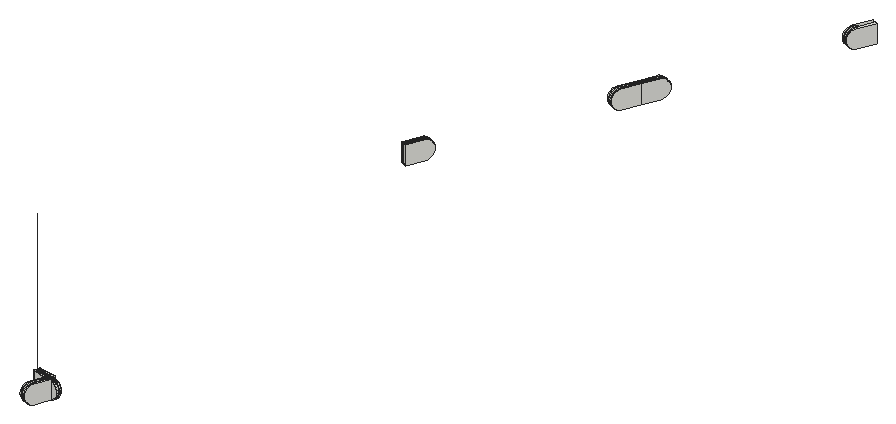
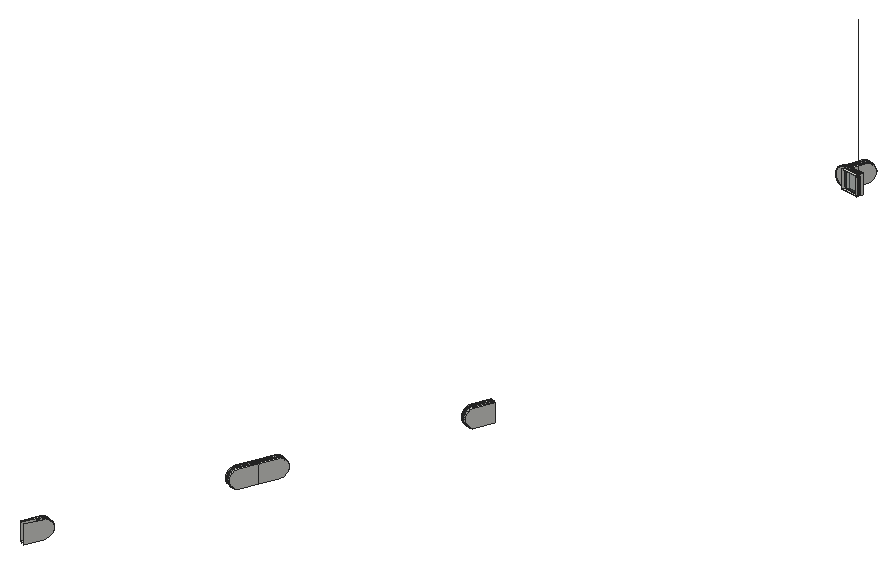
# SketchUp Ruby script. Lengths in inches.
U = 1.inch
M = Sketchup.active_model
def pt(a) = Geom::Point3d.new(a.map { |v| v * U })
def face(e, loops, mat)
  f = e.add_face(loops[0].map { |a| pt(a) })
  loops[1..].each { |l| e.add_face(l.map { |a| pt(a) }).erase! }
  f.material = f.back_material = mat if mat
  f
end
# faces: each face lists its corners as indices into pts; further lists are holes
def faces(e, pts, list, mat = nil) = list.each { |f| face(e, (f[0].is_a?(Array) ? f : [f]).map { |l| l.map { |i| pts[i] } }, mat) }
# xy, xz, yz: faces in a plane at the given z, y or x. An outline is a flat list of corners, or four numbers for a rectangle; further outlines are holes
def ring(l) = l.size == 4 ? [[l[0], l[1]], [l[2], l[1]], [l[2], l[3]], [l[0], l[3]]] : l.each_slice(2).to_a
def flat(e, list, mat, &to3) = list.each { |f| face(e, (f[0].is_a?(Array) ? f : [f]).map { |l| ring(l).map { |u, v| to3.(u, v) } }, mat) }
def xy(e, z, list, mat = nil) = flat(e, list, mat) { |x, y| [x, y, z] }
def xz(e, y, list, mat = nil) = flat(e, list, mat) { |x, z| [x, y, z] }
def yz(e, x, list, mat = nil) = flat(e, list, mat) { |y, z| [x, y, z] }
def lines(e, pts, list) = list.each { |a, b| e.add_line(pt(pts[a]), pt(pts[b])) }
# prism: a flat outline (further loops are holes) pulled along v
def prism(e, loops, v, mat = nil)
  f = face(e, loops, mat); d = Geom::Vector3d.new(v.map { |x| x * U })
  f.pushpull(f.normal.samedirection?(d) ? d.length : -d.length)
end
def box(e, o, s, mat = nil) = prism(e, [[o, [o[0] + s[0], o[1], o[2]], [o[0] + s[0], o[1] + s[1], o[2]], [o[0], o[1] + s[1], o[2]]]], [0, 0, s[2]], mat)
def at(x, y, z, deg = 0) = Geom::Transformation.translation(pt([x, y, z])) * Geom::Transformation.rotation(ORIGIN, Z_AXIS, deg.degrees)
def axes(o, x, y, z) = Geom::Transformation.new([*x, 0, *y, 0, *z, 0, *pt(o).to_a, 1])
def part(name) = M.definitions.add(name)
# library, detail: a bought-in or finely detailed component or shape, given as its bounding box
def library(name, o, s) = part(name).tap { |d| box(d.entities, o, s) }
def detail(e, o, s) = box(e.add_group.entities, o, s)
def put(e, d, t, mat = nil) = e.add_instance(d, t).tap { |i| i.material = mat if mat }
def group(e, t, mat = nil) = e.add_group.tap { |g| g.transformation = t; g.material = mat if mat }.entities
root = M.entities
M.materials.add("Glass_Safety_01").color = [204, 235, 244]
M.materials["Glass_Safety_01"].alpha = 0.1
xy(root,333,[[982.07,855.32,981.8125,855.42,981.87,855.57,982.41,856.91,982.49,856.9,982.52,857.09,982.53,857.17,982.54,857.23,982.55,857.25,982.8,857.14],[981.63,855.49,981.375,855.6,981.93,856.98,982.21,856.94],[982.49,856.9,982.41,856.91,982.49,857.1,982.52,857.09],[982.4,856.91,982.21,856.94,982.29,857.13,982.43,857.11],[982.4,856.91,982.43,857.11,982.49,857.1,982.41,856.91],
  [982.21,856.94,981.93,856.98,982.01,857.17,982.29,857.13],[981.93,856.98,980.54,857.18,980.57,857.38,982.01,857.17],[982.52,857.09,982.49,857.1,982.52,857.17,982.53,857.17],[982.49,857.1,982.43,857.11,982.44,857.1875,982.52,857.17],[982.43,857.11,982.29,857.13,982.32,857.2,982.44,857.1875],
  [982.29,857.13,982.01,857.17,982.04,857.24,982.32,857.2],[982.01,857.17,980.57,857.38,980.58,857.46,982.04,857.24],[982.52,857.17,982.44,857.1875,982.32,857.2,982.36,857.32,982.11,857.42,982.04,857.24,980.58,857.46,980.61,857.65,980.63,857.65,980.65,857.64,980.65,857.65,982.47,857.38,982.56,857.37,982.54,857.23],[982.52,857.17,982.54,857.23,982.53,857.17],[980.54,857.18,980.45,857.2,980.47,857.34,980.54,857.46,980.58,857.46,980.57,857.38],
  [982.32,857.2,982.04,857.24,982.11,857.42,982.36,857.32],[980.47,857.34,980.49,857.47,980.54,857.46],[982.47,857.38,980.65,857.65,980.78,857.88,980.72,857.91,982.51,857.65],[980.65,857.64,980.63,857.65,980.65,857.65],[980.61,857.65,980.52,857.66,980.53,857.71,980.63,857.65],
  [980.63,857.65,980.53,857.71,980.5625,857.9375,980.72,857.91,980.78,857.88,980.65,857.65],[980.73,910.8,980.48,910.91,981.27,912.72,981.52,912.61],[980.3,910.99,980.05,911.1,980.83,912.91,981.08,912.8],[989.59,931.14,989.34,931.25,989.4,931.39,990.12,933.05,990.375,932.94],[989.16,931.33,988.9,931.4375,989.6875,933.24,989.94,933.13,989.22,931.47],
  [990.375,932.94,990.12,933.05,990.91,934.86,991.16,934.75],[989.94,933.13,989.6875,933.24,990.47,935.05,990.73,934.9375],[999.21,953.22,998.95,953.33,999.02,953.48,999.74,955.13,999.99,955.02]])
xy(root,333.08,[[981.96,855.79,981.78,855.86,982.32,857.2,982.44,857.1875,982.46,857.28,982.55,857.25],[982.44,857.1875,982.32,857.2,982.36,857.32,982.46,857.28],[982.32,857.2,982.14,857.23,982.17,857.42,982.47,857.38,982.46,857.28,982.36,857.32],[982.14,857.23,980.88,857.41,980.91,857.61,982.17,857.42],[980.88,857.41,980.58,857.46,980.6,857.55,980.65,857.64,980.63,857.65,980.91,857.61],
  [980.6,857.55,980.61,857.65,980.63,857.65,980.65,857.64],[980.48,910.91,980.3,910.99,980.93,912.43,981.11,912.36],[989.49,931.61,989.3125,931.6875,989.94,933.13,990.12,933.05],[990.12,933.05,989.94,933.13,990.57,934.57,990.75,934.5]],"Glass_Safety_01")
xy(root,335.05,[[981.96,855.79,982.55,857.25,982.46,857.28,982.44,857.1875,982.32,857.2,981.78,855.86],[982.44,857.1875,982.46,857.28,982.36,857.32,982.32,857.2],[982.32,857.2,982.36,857.32,982.46,857.28,982.47,857.38,982.17,857.42,982.14,857.23],[982.14,857.23,982.17,857.42,980.91,857.61,980.88,857.41],[980.88,857.41,980.91,857.61,980.63,857.65,980.65,857.64,980.6,857.55,980.58,857.46],
  [980.6,857.55,980.65,857.64,980.63,857.65,980.61,857.65],[980.48,910.91,981.11,912.36,980.93,912.43,980.3,910.99],[989.49,931.61,990.12,933.05,989.94,933.13,989.3125,931.6875],[990.12,933.05,990.75,934.5,990.57,934.57,989.94,933.13]],"Glass_Safety_01")
xy(root,335.125,[[982.07,855.32,982.8,857.14,982.55,857.25,982.54,857.23,982.53,857.17,982.52,857.09,982.49,856.9,982.41,856.91,981.87,855.57,981.8125,855.42],[981.63,855.49,982.21,856.94,981.93,856.98,981.375,855.6],[982.49,856.9,982.52,857.09,982.49,857.1,982.41,856.91],[982.4,856.91,982.43,857.11,982.29,857.13,982.21,856.94],[982.4,856.91,982.41,856.91,982.49,857.1,982.43,857.11],
  [982.21,856.94,982.29,857.13,982.01,857.17,981.93,856.98],[981.93,856.98,982.01,857.17,980.57,857.38,980.54,857.18],[982.52,857.09,982.53,857.17,982.52,857.17,982.49,857.1],[982.49,857.1,982.52,857.17,982.44,857.1875,982.43,857.11],[982.43,857.11,982.44,857.1875,982.32,857.2,982.29,857.13],
  [982.29,857.13,982.32,857.2,982.04,857.24,982.01,857.17],[982.01,857.17,982.04,857.24,980.58,857.46,980.57,857.38],[982.52,857.17,982.54,857.23,982.56,857.37,982.47,857.38,980.65,857.65,980.65,857.64,980.63,857.65,980.61,857.65,980.58,857.46,982.04,857.24,982.11,857.42,982.36,857.32,982.32,857.2,982.44,857.1875],[982.52,857.17,982.53,857.17,982.54,857.23],[980.54,857.18,980.57,857.38,980.58,857.46,980.54,857.46,980.47,857.34,980.45,857.2],
  [982.32,857.2,982.36,857.32,982.11,857.42,982.04,857.24],[980.47,857.34,980.54,857.46,980.49,857.47],[982.47,857.38,982.51,857.65,980.72,857.91,980.78,857.88,980.65,857.65],[980.65,857.64,980.65,857.65,980.63,857.65],[980.61,857.65,980.63,857.65,980.53,857.71,980.52,857.66],
  [980.63,857.65,980.65,857.65,980.78,857.88,980.72,857.91,980.5625,857.9375,980.53,857.71],[980.73,910.8,981.52,912.61,981.27,912.72,980.48,910.91],[980.3,910.99,981.08,912.8,980.83,912.91,980.05,911.1],[989.59,931.14,990.375,932.94,990.12,933.05,989.4,931.39,989.34,931.25],[989.16,931.33,989.22,931.47,989.94,933.13,989.6875,933.24,988.9,931.4375],
  [990.375,932.94,991.16,934.75,990.91,934.86,990.12,933.05],[989.94,933.13,990.73,934.9375,990.47,935.05,989.6875,933.24],[999.21,953.22,999.99,955.02,999.74,955.13,999.02,953.48,998.95,953.33]])
yz(root,980.52,[[857.66,333,857.67,335.125]])
yz(root,980.52,[[857.66,335.125,857.67,335.125,857.67,351.28],[857.66,335.125,857.67,351.28,857.66,351.28]],"Glass_Safety_01")
p = [[982.8,857.14,335.125],[982.07,855.32,335.125],[981.97,855.0625,335.09],[981.87,854.82,334.98],[981.79,854.62,334.8125],[981.72,854.46,334.59],
  [981.68,854.36,334.34],[981.67,854.33,334.0625],[981.68,854.36,333.79],[981.72,854.46,333.53],[981.79,854.62,333.3125],[981.87,854.82,333.14],
  [981.97,855.0625,333.04],[982.07,855.32,333],[982.8,857.14,333],[981.8125,855.42,335.125],[981.87,855.57,335.125],[981.87,855.57,333],
  [981.8125,855.42,333],[981.71,855.16,333.04],[981.61,854.93,333.14],[981.53,854.72,333.3125],[981.47,854.57,333.53],[981.43,854.47,333.79],
  [981.42,854.43,334.0625],[981.43,854.47,334.34],[981.47,854.57,334.59],[981.53,854.72,334.8125],[981.61,854.93,334.98],[981.71,855.16,335.09],
  [981.63,855.49,333],[981.69,855.64,333],[981.69,855.64,335.125],[981.63,855.49,335.125],[981.53,855.24,335.09],[981.43,855,334.98],
  [981.35,854.8,334.8125],[981.29,854.64,334.59],[981.25,854.54,334.34],[981.23,854.51,334.0625],[981.25,854.54,333.79],[981.29,854.64,333.53],
  [981.35,854.8,333.3125],[981.43,855,333.14],[981.53,855.24,333.04],[982.04,857.24,335.125],[982.11,857.42,335.125],[982.11,857.42,333],
  [982.04,857.24,333],[982.01,857.17,333],[981.93,856.98,333],[981.375,855.6,333],[981.27,855.34,333.04],[981.18,855.1,333.14],
  [981.09,854.9,333.3125],[981.03,854.74,333.53],[980.99,854.64,333.79],[980.98,854.61,334.0625],[980.99,854.64,334.34],[981.03,854.74,334.59],
  [981.09,854.9,334.8125],[981.18,855.1,334.98],[981.27,855.34,335.09],[981.375,855.6,335.125],[981.93,856.98,335.125],[982.01,857.17,335.125],
  [982.21,856.94,335.125],[982.21,856.94,333],[982.29,857.13,333],[982.32,857.2,333],[982.36,857.32,333],[982.36,857.32,333.08],
  [982.32,857.2,333.08],[981.78,855.86,333.08],[981.78,855.86,335.05],[982.32,857.2,335.05],[982.36,857.32,335.05],[982.36,857.32,335.125],
  [982.32,857.2,335.125],[982.29,857.13,335.125],[982.41,856.91,333],[982.41,856.91,335.125],[982.49,857.1,335.125],[982.52,857.17,335.125],
  [982.54,857.23,335.125],[982.55,857.25,335.125],[982.55,857.25,335.05],[981.96,855.79,335.05],[981.96,855.79,333.08],[982.55,857.25,333.08],
  [982.55,857.25,333],[982.54,857.23,333],[982.52,857.17,333],[982.49,857.1,333],[982.4,856.91,335.125],[982.4,856.91,333],
  [982.49,856.9,333],[982.76,856.86,333.04],[983.02,856.82,333.14],[983.23,856.79,333.3125],[983.4,856.77,333.53],[983.51,856.75,333.79],
  [983.54,856.75,334.0625],[983.51,856.75,334.34],[983.4,856.77,334.59],[983.23,856.79,334.8125],[983.02,856.82,334.98],[982.76,856.86,335.09],
  [982.49,856.9,335.125],[982.79,857.06,333.04],[983.05,857.02,333.14],[980.54,857.18,335.125],[980.54,857.18,333],[980.57,857.38,335.125],
  [980.57,857.38,333],[982.43,857.11,333],[982.52,857.09,333],[983.26,856.99,333.3125],[983.43,856.96,333.53],[983.54,856.95,333.79],
  [983.57,856.94,334.0625],[983.54,856.95,334.34],[983.43,856.96,334.59],[983.26,856.99,334.8125],[983.05,857.02,334.98],[982.79,857.06,335.09],
  [982.52,857.09,335.125],[982.43,857.11,335.125],[982.44,857.1875,333],[982.44,857.1875,333.08],[982.44,857.1875,335.05],[982.44,857.1875,335.125],
  [982.53,857.17,335.125],[982.8,857.13,335.09],[983.06,857.1,334.98],[983.27,857.0625,334.8125],[983.44,857.04,334.59],[983.55,857.02,334.34],
  [983.58,857.02,334.0625],[983.55,857.02,333.79],[983.44,857.04,333.53],[983.27,857.0625,333.3125],[983.06,857.1,333.14],[982.8,857.13,333.04],
  [982.53,857.17,333],[982.56,857.37,333],[982.83,857.33,333.04],[983.09,857.29,333.14],[980.55,857.47,333],[980.55,857.47,333.08],
  [980.55,857.47,335.05],[980.55,857.47,335.125],[980.54,857.46,335.125],[980.47,857.34,335.125],[980.41,857.23,335.125],[980.41,857.23,333],
  [980.47,857.34,333],[980.54,857.46,333],[982.14,857.23,335.05],[982.14,857.23,333.08],[980.58,857.46,333],[980.58,857.46,333.08],
  [980.88,857.41,333.08],[980.88,857.41,335.05],[980.58,857.46,335.05],[980.58,857.46,335.125],[982.47,857.38,333],[982.47,857.38,333.08],
  [982.47,857.38,335.05],[982.47,857.38,335.125],[982.56,857.37,335.125],[982.83,857.33,335.09],[983.09,857.29,334.98],[983.3,857.26,334.8125],
  [983.47,857.23,334.59],[983.58,857.22,334.34],[983.61,857.21,334.0625],[983.58,857.22,333.79],[983.47,857.23,333.53],[983.3,857.26,333.3125],
  [980.63,857.65,333.08],[980.91,857.61,333.08],[982.17,857.42,333.08],[980.65,857.65,333],[980.63,857.65,333],[980.61,857.65,333],
  [980.61,857.65,333.08],[982.51,857.65,333],[982.51,857.65,335.125],[980.49,857.47,333],[980.49,857.47,335.125],[980.6,857.55,333.08],
  [980.65,857.64,333.08],[980.65,857.64,333],[980.78,857.88,333],[980.78,857.88,335.125],[980.65,857.65,335.125],[980.65,857.64,335.125],
  [980.65,857.64,335.05],[980.61,857.65,335.125],[980.52,857.66,335.125],[980.52,857.66,333],[980.61,857.65,335.05],[980.48,910.91,333],
  [980.48,910.91,333.08],[980.48,910.91,335.05],[980.48,910.91,335.125],[980.73,910.8,335.125],[980.73,910.8,333],[981.52,912.61,335.125],
  [981.52,912.61,333],[981.63,912.86,333.04],[981.73,913.09,333.14],[981.82,913.3,333.3125],[981.89,913.45,333.53],[981.93,913.55,333.79],
  [981.94,913.58,334.0625],[981.93,913.55,334.34],[981.89,913.45,334.59],[981.82,913.3,334.8125],[981.73,913.09,334.98],[981.63,912.86,335.09],
  [981.27,912.72,335.125],[981.27,912.72,333],[981.11,912.36,333.08],[981.11,912.36,335.05],[980.3,910.99,333],[981.08,912.8,333],
  [981.08,912.8,335.125],[980.3,910.99,335.125],[980.3,910.99,335.05],[980.93,912.43,335.05],[980.93,912.43,333.08],[980.3,910.99,333.08],
  [980.05,911.1,335.125],[980.83,912.91,335.125],[980.94,913.16,335.09],[981.04,913.39,334.98],[981.13,913.59,334.8125],[981.2,913.75,334.59],
  [981.24,913.85,334.34],[981.26,913.88,334.0625],[981.24,913.85,333.79],[981.2,913.75,333.53],[981.13,913.59,333.3125],[981.04,913.39,333.14],
  [980.94,913.16,333.04],[980.83,912.91,333],[980.05,911.1,333],[981.375,912.97,333.04],[981.48,913.2,333.14],[981.57,913.41,333.3125],
  [981.63,913.5625,333.53],[981.68,913.66,333.79],[981.69,913.69,334.0625],[981.68,913.66,334.34],[981.63,913.5625,334.59],[981.57,913.41,334.8125],
  [981.48,913.2,334.98],[981.375,912.97,335.09],[981.19,913.05,333.04],[981.19,913.05,335.09],[981.3,913.28,334.98],[981.38,913.48,334.8125],
  [981.45,913.64,334.59],[981.49,913.74,334.34],[981.51,913.77,334.0625],[981.49,913.74,333.79],[981.45,913.64,333.53],[981.38,913.48,333.3125],
  [981.3,913.28,333.14],[990.375,932.94,335.125],[989.59,931.14,335.125],[989.48,930.89,335.09],[989.375,930.65,334.98],[989.29,930.45,334.8125],
  [989.22,930.29,334.59],[989.18,930.2,334.34],[989.16,930.16,334.0625],[989.18,930.2,333.79],[989.22,930.29,333.53],[989.29,930.45,333.3125],
  [989.375,930.65,333.14],[989.48,930.89,333.04],[989.59,931.14,333],[990.375,932.94,333],[989.34,931.25,335.125],[989.4,931.39,335.125],
  [989.4,931.39,333],[989.34,931.25,333],[989.23,931,333.04],[989.125,930.76,333.14],[989.04,930.56,333.3125],[988.97,930.4,333.53],
  [988.93,930.31,333.79],[988.91,930.27,334.0625],[988.93,930.31,334.34],[988.97,930.4,334.59],[989.04,930.56,334.8125],[989.125,930.76,334.98],
  [989.23,931,335.09],[989.16,931.33,333],[989.22,931.47,333],[989.22,931.47,335.125],[989.16,931.33,335.125],[989.05,931.07,335.09],
  [988.94,930.84,334.98],[988.86,930.64,334.8125],[988.79,930.48,334.59],[988.75,930.38,334.34],[988.73,930.35,334.0625],[988.75,930.38,333.79],
  [988.79,930.48,333.53],[988.86,930.64,333.3125],[988.94,930.84,333.14],[989.05,931.07,333.04],[988.9,931.4375,335.125],[989.6875,933.24,335.125],
  [989.6875,933.24,333],[988.9,931.4375,333],[988.79,931.18,333.04],[988.69,930.95,333.14],[988.6,930.75,333.3125],[988.54,930.59,333.53],
  [988.49,930.5,333.79],[988.48,930.46,334.0625],[988.49,930.5,334.34],[988.54,930.59,334.59],[988.6,930.75,334.8125],[988.69,930.95,334.98],
  [988.79,931.18,335.09],[990.12,933.05,333],[990.12,933.05,335.125],[990.12,933.05,335.05],[989.49,931.61,335.05],[989.49,931.61,333.08],
  [990.12,933.05,333.08],[989.94,933.13,335.125],[989.94,933.13,333],[989.94,933.13,333.08],[989.3125,931.6875,333.08],[989.3125,931.6875,335.05],
  [989.94,933.13,335.05],[991.16,934.75,335.125],[991.16,934.75,333],[991.27,935,333.04],[991.37,935.23,333.14],[991.46,935.4375,333.3125],
  [991.53,935.59,333.53],[991.57,935.6875,333.79],[991.59,935.72,334.0625],[991.57,935.6875,334.34],[991.53,935.59,334.59],[991.46,935.4375,334.8125],
  [991.37,935.23,334.98],[991.27,935,335.09],[990.73,934.9375,333],[990.73,934.9375,335.125],[990.57,934.57,335.05],[990.57,934.57,333.08],
  [990.91,934.86,335.125],[990.91,934.86,333],[990.75,934.5,333.08],[990.75,934.5,335.05],[990.47,935.05,335.125],[990.58,935.3,335.09],
  [990.6875,935.53,334.98],[990.77,935.74,334.8125],[990.84,935.89,334.59],[990.88,935.99,334.34],[990.9,936.02,334.0625],[990.88,935.99,333.79],
  [990.84,935.89,333.53],[990.77,935.74,333.3125],[990.6875,935.53,333.14],[990.58,935.3,333.04],[990.47,935.05,333],[991.02,935.11,333.04],
  [990.84,935.1875,333.04],[990.84,935.1875,335.09],[990.94,935.42,334.98],[991.03,935.625,334.8125],[991.1,935.78,334.59],[991.14,935.88,334.34],
  [991.15,935.91,334.0625],[991.14,935.88,333.79],[991.1,935.78,333.53],[991.03,935.625,333.3125],[990.94,935.42,333.14],[991.12,935.34,333.14],
  [991.21,935.55,333.3125],[991.28,935.7,333.53],[991.32,935.8,333.79],[991.33,935.83,334.0625],[991.32,935.8,334.34],[991.28,935.7,334.59],
  [991.21,935.55,334.8125],[991.12,935.34,334.98],[991.02,935.11,335.09],[999.99,955.02,335.125],[999.21,953.22,335.125],[999.1,952.97,335.09],
  [998.99,952.73,334.98],[998.91,952.53,334.8125],[998.84,952.375,334.59],[998.8,952.28,334.34],[998.78,952.24,334.0625],[998.8,952.28,333.79],
  [998.84,952.375,333.53],[998.91,952.53,333.3125],[998.99,952.73,333.14],[999.1,952.97,333.04],[999.21,953.22,333],[999.99,955.02,333],
  [998.77,953.41,333],[998.84,953.56,333],[998.84,953.56,335.125],[998.77,953.41,335.125],[998.66,953.16,335.09],[998.56,952.92,334.98],
  [998.47,952.72,334.8125],[998.4,952.5625,334.59],[998.36,952.47,334.34],[998.35,952.43,334.0625],[998.36,952.47,333.79],[998.4,952.5625,333.53],
  [998.47,952.72,333.3125],[998.56,952.92,333.14],[998.66,953.16,333.04],[998.95,953.33,335.125],[999.02,953.48,335.125],[999.02,953.48,333],
  [998.95,953.33,333],[998.84,953.08,333.04],[998.74,952.84,333.14],[998.65,952.64,333.3125],[998.59,952.49,333.53],[998.54,952.39,333.79],
  [998.53,952.35,334.0625],[998.54,952.39,334.34],[998.59,952.49,334.59],[998.65,952.64,334.8125],[998.74,952.84,334.98],[998.84,953.08,335.09],
  [998.52,953.52,335.125],[999.31,955.32,335.125],[999.31,955.32,333],[998.52,953.52,333],[998.41,953.27,333.04],[998.31,953.03,333.14],
  [998.22,952.83,333.3125],[998.15,952.67,333.53],[998.11,952.58,333.79],[998.1,952.54,334.0625],[998.11,952.58,334.34],[998.15,952.67,334.59],
  [998.22,952.83,334.8125],[998.31,953.03,334.98],[998.41,953.27,335.09],[982.17,857.42,335.05],[982.46,857.28,333.08],[982.46,857.28,335.05],
  [980.91,857.61,335.05],[980.6,857.55,335.05],[980.63,857.65,335.05],[999.11,953.69,333.08],[999.11,953.69,335.05],[998.93,953.77,335.05],
  [998.93,953.77,333.08],[980.63,857.65,335.125]]
faces(root,p,[[0,1,2,3,4,5,6,7,8,9,10,11,12,13,14],[15,16,17,18,19,20,21,22,23,24,25,26,27,28,29],[30,31,32,33,34,35,36,37,38,39,40,41,42,43,44],[45,46,47,48,49,50,51,52,53,54,55,56,57,58,59,60,61,62,63,64,65],[20,19,12,11],[44,43,53,52],[19,18,13,12],[30,44,52,51],
  [66,32,31,67,68,69,70,71,72,73,74,75,76,77,78,79],[80,17,16,81,82,83,84,85,86,87,88,89,90,91,92,93],[81,94,95,80,96,97,98,99,100,101,102,103,104,105,106,107,108],[97,109,110,98],[67,95,94,66,64,111,112,50],[65,113,114,49,68,115,93,116,109,110,117,118,119,120,121,122,123,124,125,126,82,127,79],[128,129,130,131,127,94,95,115],[96,116,109,97],
  [92,128,129,130,131,83,132,133,134,135,136,137,138,139,140,141,142,143,144],[142,110,109,143],[143,109,116,144],[90,89,86,85,0,14],[145,146,143,144,91],[146,147,142,143],[148,149,150,151,152,153,154,155,156,157],[113,111,112,114],
  [78,131,130,75,158,159,72,129,128,69,48,160,161,162,163,164,165,45],[145,166,167,168,169,170,171,172,173,174,175,176,177,178,179,147,146],[71,70,47,46,77,76],[160,161,164,165,113,114],[180,181,182,167,166,183,184,185,186],[167,166,187,188,169,168],[157,189,190,152,165,164,161,160],[186,191,161,160,185],
  [192,193,183,194,195,196,197,198],[199,200,201,185,186,202],[203,204,205,206,207,208],[209,207,208,210,211,212,213,214,215,216,217,218,219,220,221],[206,222,223,203,204,224,225,205],[226,227,228,229,230,231,232,233],[234,235,236,237,238,239,240,241,242,243,244,245,246,247,248],[223,249,211,210],
  [260,227,247,246],[249,250,212,211],[270,260,246,245],[271,272,273,274,275,276,277,278,279,280,281,282,283,284,285],[286,287,288,289,290,291,292,293,294,295,296,297,298,299,300],[301,302,303,304,305,306,307,308,309,310,311,312,313,314,315],[316,317,318,319,320,321,322,323,324,325,326,327,328,329,330],[291,290,283,282],
  [315,314,321,320],[290,289,284,283],[301,315,320,319],[331,288,287,332,333,334,335,336],[337,303,302,338,339,340,341,342],[331,336,333,332,271,285],[343,271,285,344,345,346,347,348,349,350,351,352,353,354,355],[339,338,318,317,337,342],
  [338,356,357,337,342,358,359,339],[332,360,361,331,336,362,363,333],[317,364,365,366,367,368,369,370,371,372,373,374,375,376,318],[361,377,345,344],[378,356,376,375],[377,389,346,345],[388,378,375,374],[399,400,401,402,403,404,405,406,407,408,409,410,411,412,413],
  [414,415,416,417,418,419,420,421,422,423,424,425,426,427,428],[429,430,431,432,433,434,435,436,437,438,439,440,441,442,443],[444,445,446,447,448,449,450,451,452,453,454,455,456,457,458],[434,433,411,410],[428,427,449,448],[433,432,412,411],[414,428,448,447],[21,20,11,10],
  [43,42,54,53],[98,110,117,99],[141,117,110,142],[147,179,141,142],[161,164,163,162],[191,463,164,161],[250,251,213,212],[269,270,245,244],
  [292,291,282,281],[314,313,322,321],[389,390,347,346],[387,388,374,373],[435,434,410,409],[427,426,450,449],[22,21,10,9],[42,41,55,54],
  [99,117,118,100],[140,118,117,141],[179,178,140,141],[251,252,214,213],[268,269,244,243],[293,292,281,280],[313,312,323,322],[390,391,348,347],
  [386,387,373,372],[436,435,409,408],[426,425,451,450],[23,22,9,8],[41,40,56,55],[100,118,119,101],[139,119,118,140],[178,177,139,140],
  [252,253,215,214],[267,268,243,242],[294,293,280,279],[312,311,324,323],[391,392,349,348],[385,386,372,371],[437,436,408,407],[425,424,452,451],
  [24,23,8,7],[40,39,57,56],[101,119,120,102],[138,120,119,139],[177,176,138,139],[253,254,216,215],[266,267,242,241],[295,294,279,278],
  [311,310,325,324],[392,393,350,349],[384,385,371,370],[438,437,407,406],[424,423,453,452],[25,24,7,6],[39,38,58,57],[102,120,121,103],
  [137,121,120,138],[176,175,137,138],[254,255,217,216],[265,266,241,240],[296,295,278,277],[310,309,326,325],[393,394,351,350],[383,384,370,369],
  [439,438,406,405],[423,422,454,453],[26,25,6,5],[38,37,59,58],[103,121,122,104],[136,122,121,137],[175,174,136,137],[255,256,218,217],
  [264,265,240,239],[297,296,277,276],[309,308,327,326],[394,395,352,351],[382,383,369,368],[440,439,405,404],[422,421,455,454],[27,26,5,4],
  [37,36,60,59],[104,122,123,105],[135,123,122,136],[174,173,135,136],[256,257,219,218],[263,264,239,238],[298,297,276,275],[308,307,328,327],
  [395,396,353,352],[381,382,368,367],[441,440,404,403],[421,420,456,455],[28,27,4,3],[36,35,61,60],[105,123,124,106],[134,124,123,135],
  [173,172,134,135],[257,258,220,219],[262,263,238,237],[299,298,275,274],[307,306,329,328],[396,397,354,353],[380,381,367,366],[442,441,403,402],
  [420,419,457,456],[29,28,3,2],[35,34,62,61],[106,124,125,107],[133,125,124,134],[172,171,133,134],[168,459,462,464,202,199,469,196,169],[165,164,463,202,199],
  [258,259,221,220],[261,262,237,236],[300,299,274,273],[306,305,330,329],[397,398,355,354],[379,380,366,365],[443,442,402,401],[419,418,458,457],
  [15,29,2,1],[34,33,63,62],[125,107,108,126],[132,84,170,171,133,125,126],[259,222,209,221],[228,261,236,235],[286,300,273,272],[305,304,316,330],
  [398,360,343,355],[357,379,365,364],[429,443,401,400],[418,417,444,458]])
faces(root,p,[[222,223,249,250,251,252,253,254,255,256,257,258,259],[227,228,261,262,263,264,265,266,267,268,269,270,260],[356,357,379,380,381,382,383,384,385,386,387,388,378],[360,361,377,389,390,391,392,393,394,395,396,397,398],[88,87,74,73],[89,88,87,86],[72,71,76,75,74,73],[162,159,158,163],
  [158,75,130,129,72,159],[182,459,158,159],[460,461,130,129],[89,460,461,86],[76,461,460,71],[461,460,167,168],[181,162,163,462],[182,181,462,459],
  [167,182,459,168],[191,463,150,149],[463,191,192,198],[191,186,202,463],[464,462,181,180,186,202],[224,204,205,225],[233,232,231,230],[225,224,232,231],
  [335,334,341,340],[336,335,334,333],[340,339,342,341],[342,333,336,339],[339,359,358,342],[362,336,333,363],[363,362,359,358],[465,466,467,468]],"Glass_Safety_01")
